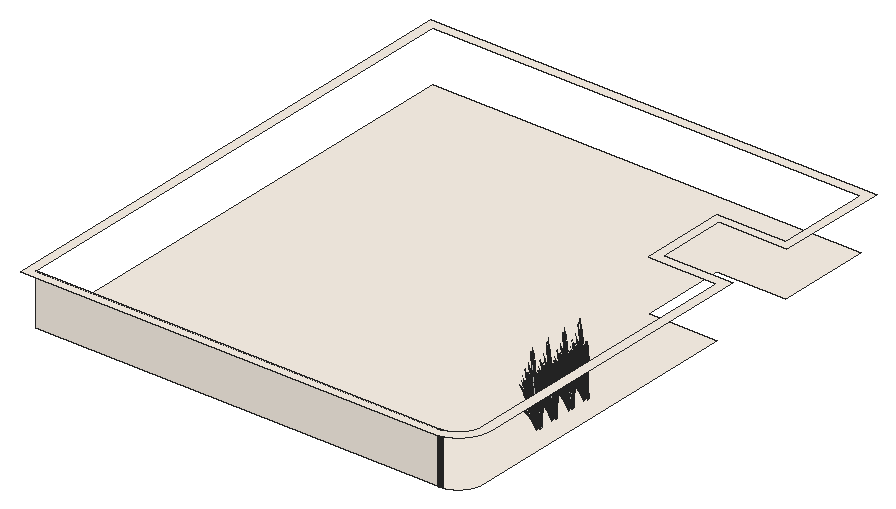
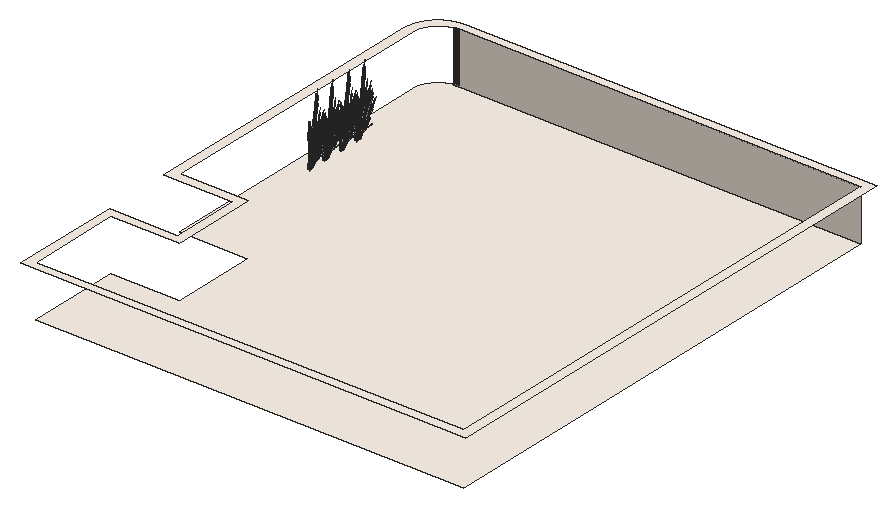
# SketchUp Ruby script. Lengths in inches.
U = 1.inch
M = Sketchup.active_model
def pt(a) = Geom::Point3d.new(a.map { |v| v * U })
def face(e, loops, mat)
  f = e.add_face(loops[0].map { |a| pt(a) })
  loops[1..].each { |l| e.add_face(l.map { |a| pt(a) }).erase! }
  f.material = f.back_material = mat if mat
  f
end
# faces: each face lists its corners as indices into pts; further lists are holes
def faces(e, pts, list, mat = nil) = list.each { |f| face(e, (f[0].is_a?(Array) ? f : [f]).map { |l| l.map { |i| pts[i] } }, mat) }
# xy, xz, yz: faces in a plane at the given z, y or x. An outline is a flat list of corners, or four numbers for a rectangle; further outlines are holes
def ring(l) = l.size == 4 ? [[l[0], l[1]], [l[2], l[1]], [l[2], l[3]], [l[0], l[3]]] : l.each_slice(2).to_a
def flat(e, list, mat, &to3) = list.each { |f| face(e, (f[0].is_a?(Array) ? f : [f]).map { |l| ring(l).map { |u, v| to3.(u, v) } }, mat) }
def xy(e, z, list, mat = nil) = flat(e, list, mat) { |x, y| [x, y, z] }
def xz(e, y, list, mat = nil) = flat(e, list, mat) { |x, z| [x, y, z] }
def yz(e, x, list, mat = nil) = flat(e, list, mat) { |y, z| [x, y, z] }
def lines(e, pts, list) = list.each { |a, b| e.add_line(pt(pts[a]), pt(pts[b])) }
# prism: a flat outline (further loops are holes) pulled along v
def prism(e, loops, v, mat = nil)
  f = face(e, loops, mat); d = Geom::Vector3d.new(v.map { |x| x * U })
  f.pushpull(f.normal.samedirection?(d) ? d.length : -d.length)
end
def box(e, o, s, mat = nil) = prism(e, [[o, [o[0] + s[0], o[1], o[2]], [o[0] + s[0], o[1] + s[1], o[2]], [o[0], o[1] + s[1], o[2]]]], [0, 0, s[2]], mat)
def at(x, y, z, deg = 0) = Geom::Transformation.translation(pt([x, y, z])) * Geom::Transformation.rotation(ORIGIN, Z_AXIS, deg.degrees)
def axes(o, x, y, z) = Geom::Transformation.new([*x, 0, *y, 0, *z, 0, *pt(o).to_a, 1])
def part(name) = M.definitions.add(name)
# library, detail: a bought-in or finely detailed component or shape, given as its bounding box
def library(name, o, s) = part(name).tap { |d| box(d.entities, o, s) }
def detail(e, o, s) = box(e.add_group.entities, o, s)
def put(e, d, t, mat = nil) = e.add_instance(d, t).tap { |i| i.material = mat if mat }
def group(e, t, mat = nil) = e.add_group.tap { |g| g.transformation = t; g.material = mat if mat }.entities
root = M.entities
M.materials.add("C01_Vanilla_Cream").color = [255, 246, 235]
M.materials.add("LightPink_Translucent").color = [144, 107, 117]
M.materials["LightPink_Translucent"].alpha = 0.75
c1 = part("blade")
p = [[2.15,0.21,22],[0,0.17,0],[0.09,0.45,0],[2.18,0.31,22],[2.29,0.31,22],[0.38,0.45,0],
  [2.48,0.24,33],[2.49,0.24,33],[2.48,0.22,33]]
faces(c1.entities,p,[[0,1,2,3],[4,5,2,3],[6,3,4,7],[8,0,3,6]])
c2 = part("seeds")
p = [[0.3,-0.1,1.38],[-0.01,-0.03,1.59],[-0.01,-0.03,0.03],[0.14,-0.07,-0.07],[0.29,-0.03,3],[0.15,0.01,3.11]]
faces(c2.entities,p,[[0,1,2,3],[1,0,4,5]],"LightPink_Translucent")
c3 = part("blade with seeds")
put(c3.entities,c1,at(0,0,0))
put(c3.entities,c2,axes([2.4,0.25,30.99],[1.5799,-0.05474,1.17369],[-0.12525,1.92788,0.29478],[-0.07173,-0.02425,1.56792]))
xy(root,654,[[54,12,336,12,336.57,12.01,337.13,12.04,337.69,12.08,338.26,12.14,338.82,12.22,339.37,12.32,339.93,12.43,340.48,12.57,341.02,12.71,341.5625,12.88,342.1,13.0625,342.625,13.26,343.15,13.48,343.66,13.71,344.17,13.96,344.67,14.23,345.16,14.51,345.64,14.8,346.12,15.11,346.58,15.4375,347.03,15.78,347.47,16.13,347.9,16.5,348.32,16.88,348.73,17.27,349.12,17.68,349.5,18.1,349.87,18.53,350.22,18.97,350.5625,19.42,350.89,19.88,351.2,20.36,351.49,20.84,351.77,21.33,352.04,21.83,352.29,22.34,352.52,22.85,352.74,23.375,352.9375,23.9,353.12,24.4375,353.29,24.98,353.43,25.52,353.57,26.07,353.68,26.63,353.78,27.18,353.86,27.74,353.92,28.31,353.96,28.87,353.99,29.43,354,30,354,234,306,234,306,294,354,294,354,360,54,360]],"C01_Vanilla_Cream")
xy(root,690,[[[48,6,336,6,336.75,6.01,337.51,6.05,338.26,6.11,339.01,6.1875,339.75,6.3,340.5,6.43,341.24,6.58,341.97,6.75,342.7,6.95,343.42,7.17,344.13,7.42,344.83,7.69,345.53,7.97,346.22,8.28,346.9,8.62,347.5625,8.97,348.22,9.34,348.86,9.74,349.49,10.15,350.11,10.58,350.71,11.04,351.3,11.51,351.87,12,352.43,12.5,352.97,13.03,353.5,13.57,354,14.13,354.49,14.7,354.96,15.29,355.42,15.89,355.85,16.51,356.26,17.14,356.66,17.78,357.03,18.4375,357.38,19.1,357.72,19.78,358.03,20.47,358.31,21.17,358.58,21.87,358.83,22.58,359.05,23.3,359.25,24.03,359.42,24.76,359.57,25.5,359.7,26.25,359.8125,26.99,359.89,27.74,359.95,28.49,359.99,29.25,360,30,360,240,312,240,312,288,360,288,360,366,48,366],[54,12,54,360,354,360,354,294,306,294,306,234,354,234,354,30,353.99,29.43,353.96,28.87,353.92,28.31,353.86,27.74,353.78,27.18,353.68,26.63,353.57,26.07,353.43,25.52,353.29,24.98,353.12,24.4375,352.9375,23.9,352.74,23.375,352.52,22.85,352.29,22.34,352.04,21.83,351.77,21.33,351.49,20.84,351.2,20.36,350.89,19.88,350.5625,19.42,350.22,18.97,349.87,18.53,349.5,18.1,349.12,17.68,348.73,17.27,348.32,16.88,347.9,16.5,347.47,16.13,347.03,15.78,346.58,15.4375,346.12,15.11,345.64,14.8,345.16,14.51,344.67,14.23,344.17,13.96,343.66,13.71,343.15,13.48,342.625,13.26,342.1,13.0625,341.5625,12.88,341.02,12.71,340.48,12.57,339.93,12.43,339.37,12.32,338.82,12.22,338.26,12.14,337.69,12.08,337.13,12.04,336.57,12.01,336,12]]],"C01_Vanilla_Cream")
xz(root,12,[[54,654,336,690]],"C01_Vanilla_Cream")
p = [[336.57,12.01,654],[336,12,654],[336,12,690],[336.57,12.01,690],[337.13,12.04,654],[337.13,12.04,690],
  [337.69,12.08,654],[337.69,12.08,690],[338.26,12.14,654],[338.26,12.14,690],[338.82,12.22,654],[338.82,12.22,690],
  [339.37,12.32,654],[339.37,12.32,690]]
faces(root,p,[[0,1,2,3],[4,0,3,5],[6,4,5,7],[8,6,7,9],[10,8,9,11],[12,10,11,13]],"C01_Vanilla_Cream")
put(root,c3,axes([339.83,94.1,657.18],[0.20495,-0.00938,1.40529],[-0.13596,0.40664,0.11363],[-0.29207,-0.02515,0.60075]))
put(root,c3,axes([339.83,107.7,657.18],[0.20495,-0.00938,1.40529],[-0.13596,0.40664,0.11363],[-0.29207,-0.02515,0.60075]))
put(root,c3,axes([339.83,122.09,657.18],[0.20495,-0.00938,1.40529],[-0.13596,0.40664,0.11363],[-0.29207,-0.02515,0.60075]))
put(root,c3,axes([339.83,135.58,657.18],[0.20495,-0.00938,1.40529],[-0.13596,0.40664,0.11363],[-0.29207,-0.02515,0.60075]))
put(root,c3,axes([339.92,94.81,657.18],[0.17145,-0.08763,1.40529],[0.14434,0.4049,0.11363],[-0.26915,0.09151,0.60075]))
put(root,c3,axes([339.92,108.41,657.18],[0.17145,-0.08763,1.40529],[0.14434,0.4049,0.11363],[-0.26915,0.09151,0.60075]))
put(root,c3,axes([339.92,122.81,657.18],[0.17145,-0.08763,1.40529],[0.14434,0.4049,0.11363],[-0.26915,0.09151,0.60075]))
put(root,c3,axes([339.92,136.3,657.18],[0.17145,-0.08763,1.40529],[0.14434,0.4049,0.11363],[-0.26915,0.09151,0.60075]))
put(root,c3,axes([339.39,95.5,656.125],[0.17172,0.03401,1.17261],[0.11068,0.34736,-0.25218],[-0.23326,0.06502,0.50135]))
put(root,c3,axes([339.39,109.1,656.125],[0.17172,0.03401,1.17261],[0.11068,0.34736,-0.25218],[-0.23326,0.06502,0.50135]))
put(root,c3,axes([339.39,123.5,656.125],[0.17172,0.03401,1.17261],[0.11068,0.34736,-0.25218],[-0.23326,0.06502,0.50135]))
put(root,c3,axes([339.39,136.99,656.125],[0.17172,0.03401,1.17261],[0.11068,0.34736,-0.25218],[-0.23326,0.06502,0.50135]))
put(root,c3,axes([340.9,94.39,656.74],[0.14045,-0.05993,1.45192],[0.04843,0.41842,0.11363],[-0.30422,0.05552,0.51893]))
put(root,c3,axes([340.9,107.99,656.74],[0.14045,-0.05993,1.45192],[0.04843,0.41842,0.11363],[-0.30422,0.05552,0.51893]))
put(root,c3,axes([340.9,122.39,656.74],[0.14045,-0.05993,1.45192],[0.04843,0.41842,0.11363],[-0.30422,0.05552,0.51893]))
put(root,c3,axes([340.9,135.875,656.74],[0.14045,-0.05993,1.45192],[0.04843,0.41842,0.11363],[-0.30422,0.05552,0.51893]))
put(root,c3,axes([339.39,94.67,657.87],[-0.08069,0.05378,1.43454],[0.00686,0.39297,-0.22687],[-0.18495,0.0511,0.11505]))
put(root,c3,axes([339.39,108.27,657.87],[-0.08069,0.05378,1.43454],[0.00686,0.39297,-0.22687],[-0.18495,0.0511,0.11505]))
put(root,c3,axes([339.39,122.67,657.87],[-0.08069,0.05378,1.43454],[0.00686,0.39297,-0.22687],[-0.18495,0.0511,0.11505]))
put(root,c3,axes([339.39,136.16,657.87],[-0.08069,0.05378,1.43454],[0.00686,0.39297,-0.22687],[-0.18495,0.0511,0.11505]))
put(root,c3,axes([340.45,93.72,658.08],[-0.49394,-0.00997,-0.58257],[0.03317,-0.42002,0.0703],[-0.20925,-0.04433,0.8241]))
put(root,c3,axes([340.45,107.32,658.08],[-0.49394,-0.00997,-0.58257],[0.03317,-0.42002,0.0703],[-0.20925,-0.04433,0.8241]))
put(root,c3,axes([340.45,121.72,658.08],[-0.49394,-0.00997,-0.58257],[0.03317,-0.42002,0.0703],[-0.20925,-0.04433,0.8241]))
put(root,c3,axes([340.45,135.21,658.08],[-0.49394,-0.00997,-0.58257],[0.03317,-0.42002,0.0703],[-0.20925,-0.04433,0.8241]))
put(root,c3,axes([340.05,93.82,656.125],[0.09647,0.11534,1.17261],[-0.2223,0.31351,-0.25218],[-0.22826,-0.07493,0.50135]))
put(root,c3,axes([340.05,107.42,656.125],[0.09647,0.11534,1.17261],[-0.2223,0.31351,-0.25218],[-0.22826,-0.07493,0.50135]))
put(root,c3,axes([340.05,121.82,656.125],[0.09647,0.11534,1.17261],[-0.2223,0.31351,-0.25218],[-0.22826,-0.07493,0.50135]))
put(root,c3,axes([340.05,135.31,656.125],[0.09647,0.11534,1.17261],[-0.2223,0.31351,-0.25218],[-0.22826,-0.07493,0.50135]))
put(root,c3,axes([339.65,94.45,657.71],[-0.41064,-0.11557,-0.29039],[0.11977,-0.33716,0.3749],[-0.16533,0.03092,0.71734]))
put(root,c3,axes([339.65,108.05,657.71],[-0.41064,-0.11557,-0.29039],[0.11977,-0.33716,0.3749],[-0.16533,0.03092,0.71734]))
put(root,c3,axes([339.65,122.44,657.71],[-0.41064,-0.11557,-0.29039],[0.11977,-0.33716,0.3749],[-0.16533,0.03092,0.71734]))
put(root,c3,axes([339.65,135.93,657.71],[-0.41064,-0.11557,-0.29039],[0.11977,-0.33716,0.3749],[-0.16533,0.03092,0.71734]))
put(root,c3,axes([340.22,93.45,657.18],[0.18354,0.07137,1.40529],[-0.37983,0.29943,0.11363],[-0.23673,-0.13508,0.60075]))
put(root,c3,axes([340.22,107.05,657.18],[0.18354,0.07137,1.40529],[-0.37983,0.29943,0.11363],[-0.23673,-0.13508,0.60075]))
put(root,c3,axes([340.22,121.44,657.18],[0.18354,0.07137,1.40529],[-0.37983,0.29943,0.11363],[-0.23673,-0.13508,0.60075]))
put(root,c3,axes([340.22,134.93,657.18],[0.18354,0.07137,1.40529],[-0.37983,0.29943,0.11363],[-0.23673,-0.13508,0.60075]))
put(root,c3,axes([338.5,95.07,657.86],[0.06306,0.01111,1.45454],[0.19508,0.36602,-0.13744],[-0.12909,0.09607,0.2574]))
put(root,c3,axes([338.5,108.67,657.86],[0.06306,0.01111,1.45454],[0.19508,0.36602,-0.13744],[-0.12909,0.09607,0.2574]))
put(root,c3,axes([338.5,123.0625,657.86],[0.06306,0.01111,1.45454],[0.19508,0.36602,-0.13744],[-0.12909,0.09607,0.2574]))
put(root,c3,axes([338.5,136.55,657.86],[0.06306,0.01111,1.45454],[0.19508,0.36602,-0.13744],[-0.12909,0.09607,0.2574]))
put(root,c3,axes([339.94,94.62,657.84],[-0.13386,0.37682,-0.41901],[-0.45895,-0.12916,-0.32456],[-0.18478,0.03455,0.80174]))
put(root,c3,axes([339.94,108.22,657.84],[-0.13386,0.37682,-0.41901],[-0.45895,-0.12916,-0.32456],[-0.18478,0.03455,0.80174]))
put(root,c3,axes([339.94,122.61,657.84],[-0.13386,0.37682,-0.41901],[-0.45895,-0.12916,-0.32456],[-0.18478,0.03455,0.80174]))
put(root,c3,axes([339.94,136.1,657.84],[-0.13386,0.37682,-0.41901],[-0.45895,-0.12916,-0.32456],[-0.18478,0.03455,0.80174]))
put(root,c3,axes([340.28,93.81,657.84],[-0.35879,0.27441,-0.41901],[-0.31422,-0.28988,-0.32456],[-0.18229,-0.04175,0.80174]))
put(root,c3,axes([340.28,107.4,657.84],[-0.35879,0.27441,-0.41901],[-0.31422,-0.28988,-0.32456],[-0.18229,-0.04175,0.80174]))
put(root,c3,axes([340.28,121.8,657.84],[-0.35879,0.27441,-0.41901],[-0.31422,-0.28988,-0.32456],[-0.18229,-0.04175,0.80174]))
put(root,c3,axes([340.28,135.29,657.84],[-0.35879,0.27441,-0.41901],[-0.31422,-0.28988,-0.32456],[-0.18229,-0.04175,0.80174]))
put(root,c3,axes([339.7,94.6,655.22],[0.01253,0.06529,1.44601],[-0.25262,0.34095,-0.2209],[-0.17944,-0.01719,0.2463]))
put(root,c3,axes([339.7,108.2,655.22],[0.01253,0.06529,1.44601],[-0.25262,0.34095,-0.2209],[-0.17944,-0.01719,0.2463]))
put(root,c3,axes([339.7,122.59,655.22],[0.01253,0.06529,1.44601],[-0.25262,0.34095,-0.2209],[-0.17944,-0.01719,0.2463]))
put(root,c3,axes([339.7,136.08,655.22],[0.01253,0.06529,1.44601],[-0.25262,0.34095,-0.2209],[-0.17944,-0.01719,0.2463]))
put(root,c3,axes([339.78,93.04,657.86],[0.03663,0.04134,1.45454],[-0.17659,0.37163,-0.13744],[-0.17885,0.00269,0.2574]))
put(root,c3,axes([339.78,106.64,657.86],[0.03663,0.04134,1.45454],[-0.17659,0.37163,-0.13744],[-0.17885,0.00269,0.2574]))
put(root,c3,axes([339.78,121.03,657.86],[0.03663,0.04134,1.45454],[-0.17659,0.37163,-0.13744],[-0.17885,0.00269,0.2574]))
put(root,c3,axes([339.78,134.52,657.86],[0.03663,0.04134,1.45454],[-0.17659,0.37163,-0.13744],[-0.17885,0.00269,0.2574]))
put(root,c3,axes([339.03,96.23,656.27],[0.20592,-0.18775,0.94186],[0.08126,0.29723,0.69201],[-0.14881,0.05322,0.20745]))
put(root,c3,axes([339.03,109.83,656.27],[0.20592,-0.18775,0.94186],[0.08126,0.29723,0.69201],[-0.14881,0.05322,0.20745]))
put(root,c3,axes([339.03,124.23,656.27],[0.20592,-0.18775,0.94186],[0.08126,0.29723,0.69201],[-0.14881,0.05322,0.20745]))
put(root,c3,axes([339.03,137.72,656.27],[0.20592,-0.18775,0.94186],[0.08126,0.29723,0.69201],[-0.14881,0.05322,0.20745]))
put(root,c3,axes([340.1875,92.79,657.87],[-0.10632,-0.00292,1.43454],[-0.33847,0.29241,-0.22687],[-0.1806,-0.05975,0.11505]))
put(root,c3,axes([340.1875,106.39,657.87],[-0.10632,-0.00292,1.43454],[-0.33847,0.29241,-0.22687],[-0.1806,-0.05975,0.11505]))
put(root,c3,axes([340.1875,120.78,657.87],[-0.10632,-0.00292,1.43454],[-0.33847,0.29241,-0.22687],[-0.1806,-0.05975,0.11505]))
put(root,c3,axes([340.1875,134.27,657.87],[-0.10632,-0.00292,1.43454],[-0.33847,0.29241,-0.22687],[-0.1806,-0.05975,0.11505]))
put(root,c3,axes([339.75,94.41,657.88],[0.1396,-0.37772,0.39362],[0.45895,0.12916,0.32456],[-0.18049,0.0227,0.8145]))
put(root,c3,axes([339.75,108.01,657.88],[0.1396,-0.37772,0.39362],[0.45895,0.12916,0.32456],[-0.18049,0.0227,0.8145]))
put(root,c3,axes([339.75,122.4,657.88],[0.1396,-0.37772,0.39362],[0.45895,0.12916,0.32456],[-0.18049,0.0227,0.8145]))
put(root,c3,axes([339.75,135.89,657.88],[0.1396,-0.37772,0.39362],[0.45895,0.12916,0.32456],[-0.18049,0.0227,0.8145]))
put(root,c3,axes([339.91,94.3,658.13],[0.24861,0.37512,-0.09971],[-0.44125,0.18434,-0.55346],[-0.18594,0.04949,0.84097]))
put(root,c3,axes([339.91,107.9,658.13],[0.24861,0.37512,-0.09971],[-0.44125,0.18434,-0.55346],[-0.18594,0.04949,0.84097]))
put(root,c3,axes([339.91,122.29,658.13],[0.24861,0.37512,-0.09971],[-0.44125,0.18434,-0.55346],[-0.18594,0.04949,0.84097]))
put(root,c3,axes([339.91,135.78,658.13],[0.24861,0.37512,-0.09971],[-0.44125,0.18434,-0.55346],[-0.18594,0.04949,0.84097]))
put(root,c3,axes([340.47,93.52,658.13],[-0.02646,0.4213,-0.09971],[-0.50094,-0.01152,-0.55346],[-0.19293,-0.02926,0.84097]))
put(root,c3,axes([340.47,107.12,658.13],[-0.02646,0.4213,-0.09971],[-0.50094,-0.01152,-0.55346],[-0.19293,-0.02926,0.84097]))
put(root,c3,axes([340.47,121.51,658.13],[-0.02646,0.4213,-0.09971],[-0.50094,-0.01152,-0.55346],[-0.19293,-0.02926,0.84097]))
put(root,c3,axes([340.47,135,658.13],[-0.02646,0.4213,-0.09971],[-0.50094,-0.01152,-0.55346],[-0.19293,-0.02926,0.84097]))
put(root,c3,axes([340.15,93.55,657.71],[-0.28114,-0.25937,-0.29039],[0.32102,-0.24553,0.3749],[-0.16311,-0.03736,0.71734]))
put(root,c3,axes([340.15,107.15,657.71],[-0.28114,-0.25937,-0.29039],[0.32102,-0.24553,0.3749],[-0.16311,-0.03736,0.71734]))
put(root,c3,axes([340.15,121.54,657.71],[-0.28114,-0.25937,-0.29039],[0.32102,-0.24553,0.3749],[-0.16311,-0.03736,0.71734]))
put(root,c3,axes([340.15,135.03,657.71],[-0.28114,-0.25937,-0.29039],[0.32102,-0.24553,0.3749],[-0.16311,-0.03736,0.71734]))
put(root,c3,axes([339.71,94.31,657.88],[-0.18148,-0.28246,0.05273],[0.33093,-0.13825,0.41509],[-0.14588,0.02728,0.63295]))
put(root,c3,axes([339.71,107.9,657.88],[-0.18148,-0.28246,0.05273],[0.33093,-0.13825,0.41509],[-0.14588,0.02728,0.63295]))
put(root,c3,axes([339.71,122.3,657.88],[-0.18148,-0.28246,0.05273],[0.33093,-0.13825,0.41509],[-0.14588,0.02728,0.63295]))
put(root,c3,axes([339.71,135.79,657.88],[-0.18148,-0.28246,0.05273],[0.33093,-0.13825,0.41509],[-0.14588,0.02728,0.63295]))
put(root,c3,axes([340.55,95.09,657.18],[0.12341,-0.12729,1.40529],[0.31162,0.34357,0.11363],[-0.21373,0.15646,0.60075]))
put(root,c3,axes([340.55,108.6875,657.18],[0.12341,-0.12729,1.40529],[0.31162,0.34357,0.11363],[-0.21373,0.15646,0.60075]))
put(root,c3,axes([340.55,123.08,657.18],[0.12341,-0.12729,1.40529],[0.31162,0.34357,0.11363],[-0.21373,0.15646,0.60075]))
put(root,c3,axes([340.55,136.57,657.18],[0.12341,-0.12729,1.40529],[0.31162,0.34357,0.11363],[-0.21373,0.15646,0.60075]))
put(root,c3,axes([339.8,95.42,657.71],[-0.43011,0.0592,-0.29039],[-0.11357,-0.33844,0.3749],[-0.12326,0.0909,0.71734]))
put(root,c3,axes([339.8,109.02,657.71],[-0.43011,0.0592,-0.29039],[-0.11357,-0.33844,0.3749],[-0.12326,0.0909,0.71734]))
put(root,c3,axes([339.8,123.41,657.71],[-0.43011,0.0592,-0.29039],[-0.11357,-0.33844,0.3749],[-0.12326,0.0909,0.71734]))
put(root,c3,axes([339.8,136.91,657.71],[-0.43011,0.0592,-0.29039],[-0.11357,-0.33844,0.3749],[-0.12326,0.0909,0.71734]))
put(root,c3,axes([339.57,96.43,655.22],[0.06628,0.04139,1.44601],[0.11238,0.38347,-0.2209],[-0.14689,0.08177,0.2463]))
put(root,c3,axes([339.57,110.02,655.22],[0.06628,0.04139,1.44601],[0.11238,0.38347,-0.2209],[-0.14689,0.08177,0.2463]))
put(root,c3,axes([339.57,124.42,655.22],[0.06628,0.04139,1.44601],[0.11238,0.38347,-0.2209],[-0.14689,0.08177,0.2463]))
put(root,c3,axes([339.57,137.91,655.22],[0.06628,0.04139,1.44601],[0.11238,0.38347,-0.2209],[-0.14689,0.08177,0.2463]))
put(root,c3,axes([339.47,94.17,656.27],[0.31546,-0.02964,0.94186],[-0.20011,0.26119,0.69201],[-0.15589,-0.03918,0.20745]))
put(root,c3,axes([339.47,107.77,656.27],[0.31546,-0.02964,0.94186],[-0.20011,0.26119,0.69201],[-0.15589,-0.03918,0.20745]))
put(root,c3,axes([339.47,122.16,656.27],[0.31546,-0.02964,0.94186],[-0.20011,0.26119,0.69201],[-0.15589,-0.03918,0.20745]))
put(root,c3,axes([339.47,135.65,656.27],[0.31546,-0.02964,0.94186],[-0.20011,0.26119,0.69201],[-0.15589,-0.03918,0.20745]))
put(root,c3,axes([339.86,95.35,657.88],[-0.12254,-0.38127,0.39362],[0.48071,-0.06617,0.32456],[-0.14168,0.08967,0.8145]))
put(root,c3,axes([339.86,108.95,657.88],[-0.12254,-0.38127,0.39362],[0.48071,-0.06617,0.32456],[-0.14168,0.08967,0.8145]))
put(root,c3,axes([339.86,123.34,657.88],[-0.12254,-0.38127,0.39362],[0.48071,-0.06617,0.32456],[-0.14168,0.08967,0.8145]))
put(root,c3,axes([339.86,136.83,657.88],[-0.12254,-0.38127,0.39362],[0.48071,-0.06617,0.32456],[-0.14168,0.08967,0.8145]))
put(root,c3,axes([340.11,93.45,658.18],[0.40806,-0.30572,0.44086],[0.35193,0.32467,0.3635],[-0.19145,-0.05639,0.91224]))
put(root,c3,axes([340.11,107.05,658.18],[0.40806,-0.30572,0.44086],[0.35193,0.32467,0.3635],[-0.19145,-0.05639,0.91224]))
put(root,c3,axes([340.11,121.44,658.18],[0.40806,-0.30572,0.44086],[0.35193,0.32467,0.3635],[-0.19145,-0.05639,0.91224]))
put(root,c3,axes([340.11,134.94,658.18],[0.40806,-0.30572,0.44086],[0.35193,0.32467,0.3635],[-0.19145,-0.05639,0.91224]))
put(root,c3,axes([339.76,95.27,657.88],[-0.33921,-0.17422,0.05273],[0.19749,-0.2481,0.41509],[-0.10876,0.08021,0.63295]))
put(root,c3,axes([339.76,108.87,657.88],[-0.33921,-0.17422,0.05273],[0.19749,-0.2481,0.41509],[-0.10876,0.08021,0.63295]))
put(root,c3,axes([339.76,123.27,657.88],[-0.33921,-0.17422,0.05273],[0.19749,-0.2481,0.41509],[-0.10876,0.08021,0.63295]))
put(root,c3,axes([339.76,136.76,657.88],[-0.33921,-0.17422,0.05273],[0.19749,-0.2481,0.41509],[-0.10876,0.08021,0.63295]))
put(root,c3,axes([340.45,95.4,657.18],[0.092,-0.14239,1.40529],[0.38596,0.29467,0.11363],[-0.17411,0.18366,0.60075]))
put(root,c3,axes([340.45,109,657.18],[0.092,-0.14239,1.40529],[0.38596,0.29467,0.11363],[-0.17411,0.18366,0.60075]))
put(root,c3,axes([340.45,123.4,657.18],[0.092,-0.14239,1.40529],[0.38596,0.29467,0.11363],[-0.17411,0.18366,0.60075]))
put(root,c3,axes([340.09,94.41,658.14],[0.41064,0.11557,0.29039],[-0.11977,0.33716,-0.3749],[-0.16533,0.03092,0.71734]))
put(root,c3,axes([340.09,108.01,658.14],[0.41064,0.11557,0.29039],[-0.11977,0.33716,-0.3749],[-0.16533,0.03092,0.71734]))
put(root,c3,axes([340.09,122.41,658.14],[0.41064,0.11557,0.29039],[-0.11977,0.33716,-0.3749],[-0.16533,0.03092,0.71734]))
put(root,c3,axes([340.09,135.9,658.14],[0.41064,0.11557,0.29039],[-0.11977,0.33716,-0.3749],[-0.16533,0.03092,0.71734]))
put(root,c3,axes([340.16,95.46,657.84],[0.12693,0.37826,-0.41901],[-0.48071,0.06617,-0.32456],[-0.13776,0.1016,0.80174]))
put(root,c3,axes([340.16,109.06,657.84],[0.12693,0.37826,-0.41901],[-0.48071,0.06617,-0.32456],[-0.13776,0.1016,0.80174]))
put(root,c3,axes([340.16,123.45,657.84],[0.12693,0.37826,-0.41901],[-0.48071,0.06617,-0.32456],[-0.13776,0.1016,0.80174]))
put(root,c3,axes([340.16,136.94,657.84],[0.12693,0.37826,-0.41901],[-0.48071,0.06617,-0.32456],[-0.13776,0.1016,0.80174]))
put(root,c3,axes([340.29,93.45,657.88],[0.02488,-0.31501,0.05273],[0.3757,0.00864,0.41509],[-0.14392,-0.03296,0.63295]))
put(root,c3,axes([340.29,107.05,657.88],[0.02488,-0.31501,0.05273],[0.3757,0.00864,0.41509],[-0.14392,-0.03296,0.63295]))
put(root,c3,axes([340.29,121.44,657.88],[0.02488,-0.31501,0.05273],[0.3757,0.00864,0.41509],[-0.14392,-0.03296,0.63295]))
put(root,c3,axes([340.29,134.93,657.88],[0.02488,-0.31501,0.05273],[0.3757,0.00864,0.41509],[-0.14392,-0.03296,0.63295]))
put(root,c3,axes([339.41,96.14,657.87],[-0.01228,0.08198,1.43454],[0.34856,0.28519,-0.22687],[-0.09125,0.13486,0.11505]))
put(root,c3,axes([339.41,109.74,657.87],[-0.01228,0.08198,1.43454],[0.34856,0.28519,-0.22687],[-0.09125,0.13486,0.11505]))
put(root,c3,axes([339.41,124.13,657.87],[-0.01228,0.08198,1.43454],[0.34856,0.28519,-0.22687],[-0.09125,0.13486,0.11505]))
put(root,c3,axes([341.36,95.1875,655.6875],[-0.514,-0.06792,-0.51129],[0.10846,-0.41895,-0.13419],[-0.15339,-0.05076,1.12859]))
put(root,c3,axes([341.36,108.79,655.6875],[-0.514,-0.06792,-0.51129],[0.10846,-0.41895,-0.13419],[-0.15339,-0.05076,1.12859]))
put(root,c3,axes([341.36,123.18,655.6875],[-0.514,-0.06792,-0.51129],[0.10846,-0.41895,-0.13419],[-0.15339,-0.05076,1.12859]))
put(root,c3,axes([341.36,136.67,655.6875],[-0.514,-0.06792,-0.51129],[0.10846,-0.41895,-0.13419],[-0.15339,-0.05076,1.12859]))
put(root,c3,axes([341.45,92.9,658.45],[-0.32977,0.39714,-0.11168],[-0.47757,-0.2288,-0.61987],[-0.16601,-0.1122,0.94188]))
put(root,c3,axes([341.45,106.5,658.45],[-0.32977,0.39714,-0.11168],[-0.47757,-0.2288,-0.61987],[-0.16601,-0.1122,0.94188]))
put(root,c3,axes([341.45,120.9,658.45],[-0.32977,0.39714,-0.11168],[-0.47757,-0.2288,-0.61987],[-0.16601,-0.1122,0.94188]))
put(root,c3,axes([341.45,134.39,658.45],[-0.32977,0.39714,-0.11168],[-0.47757,-0.2288,-0.61987],[-0.16601,-0.1122,0.94188]))
put(root,c3,axes([340.55,93.68,658.14],[0.28114,0.25937,0.29039],[-0.32102,0.24553,-0.3749],[-0.16311,-0.03736,0.71734]))
put(root,c3,axes([340.55,107.28,658.14],[0.28114,0.25937,0.29039],[-0.32102,0.24553,-0.3749],[-0.16311,-0.03736,0.71734]))
put(root,c3,axes([340.55,121.68,658.14],[0.28114,0.25937,0.29039],[-0.32102,0.24553,-0.3749],[-0.16311,-0.03736,0.71734]))
put(root,c3,axes([340.55,135.17,658.14],[0.28114,0.25937,0.29039],[-0.32102,0.24553,-0.3749],[-0.16311,-0.03736,0.71734]))
put(root,c3,axes([341.31,93.23,658.08],[-0.42133,-0.20023,-0.58257],[0.29943,-0.35088,0.0703],[-0.15265,-0.11956,0.8241]))
put(root,c3,axes([341.31,106.82,658.08],[-0.42133,-0.20023,-0.58257],[0.29943,-0.35088,0.0703],[-0.15265,-0.11956,0.8241]))
put(root,c3,axes([341.31,121.22,658.08],[-0.42133,-0.20023,-0.58257],[0.29943,-0.35088,0.0703],[-0.15265,-0.11956,0.8241]))
put(root,c3,axes([341.31,134.71,658.08],[-0.42133,-0.20023,-0.58257],[0.29943,-0.35088,0.0703],[-0.15265,-0.11956,0.8241]))
put(root,c3,axes([341.11,93.24,657.84],[-0.48758,0.09847,-0.41901],[-0.08529,-0.37293,-0.32456],[-0.13096,-0.10687,0.80174]))
put(root,c3,axes([341.11,106.83,657.84],[-0.48758,0.09847,-0.41901],[-0.08529,-0.37293,-0.32456],[-0.13096,-0.10687,0.80174]))
put(root,c3,axes([341.11,121.23,657.84],[-0.48758,0.09847,-0.41901],[-0.08529,-0.37293,-0.32456],[-0.13096,-0.10687,0.80174]))
put(root,c3,axes([341.11,134.72,657.84],[-0.48758,0.09847,-0.41901],[-0.08529,-0.37293,-0.32456],[-0.13096,-0.10687,0.80174]))
put(root,c3,axes([340.68,95.98,655.65],[-0.46245,-0.20713,-0.40713],[0.27641,-0.37142,0],[-0.10533,-0.04718,1.29153]))
put(root,c3,axes([340.68,109.58,655.65],[-0.46245,-0.20713,-0.40713],[0.27641,-0.37142,0],[-0.10533,-0.04718,1.29153]))
put(root,c3,axes([340.68,123.98,655.65],[-0.46245,-0.20713,-0.40713],[0.27641,-0.37142,0],[-0.10533,-0.04718,1.29153]))
put(root,c3,axes([340.68,137.47,655.65],[-0.46245,-0.20713,-0.40713],[0.27641,-0.37142,0],[-0.10533,-0.04718,1.29153]))
put(root,c3,axes([340.48,92.9,655.22],[-0.04786,0.05457,1.44601],[-0.48369,0.11766,-0.2209],[-0.11685,-0.10703,0.2463]))
put(root,c3,axes([340.48,106.5,655.22],[-0.04786,0.05457,1.44601],[-0.48369,0.11766,-0.2209],[-0.11685,-0.10703,0.2463]))
put(root,c3,axes([340.48,120.89,655.22],[-0.04786,0.05457,1.44601],[-0.48369,0.11766,-0.2209],[-0.11685,-0.10703,0.2463]))
put(root,c3,axes([340.48,134.38,655.22],[-0.04786,0.05457,1.44601],[-0.48369,0.11766,-0.2209],[-0.11685,-0.10703,0.2463]))
put(root,c3,axes([339.93,95.19,658.13],[0.45707,0.22842,-0.09971],[-0.26332,0.3308,-0.55346],[-0.12913,0.11499,0.84097]))
put(root,c3,axes([339.93,108.79,658.13],[0.45707,0.22842,-0.09971],[-0.26332,0.3308,-0.55346],[-0.12913,0.11499,0.84097]))
put(root,c3,axes([339.93,123.18,658.13],[0.45707,0.22842,-0.09971],[-0.26332,0.3308,-0.55346],[-0.12913,0.11499,0.84097]))
put(root,c3,axes([339.93,136.67,658.13],[0.45707,0.22842,-0.09971],[-0.26332,0.3308,-0.55346],[-0.12913,0.11499,0.84097]))
put(root,c3,axes([340.96,96.23,655.95],[-0.30893,0.41511,0],[-0.51685,-0.2315,-0.42318],[-0.11772,-0.05273,1.34243]))
put(root,c3,axes([340.96,109.83,655.95],[-0.30893,0.41511,0],[-0.51685,-0.2315,-0.42318],[-0.11772,-0.05273,1.34243]))
put(root,c3,axes([340.96,124.23,655.95],[-0.30893,0.41511,0],[-0.51685,-0.2315,-0.42318],[-0.11772,-0.05273,1.34243]))
put(root,c3,axes([340.96,137.72,655.95],[-0.30893,0.41511,0],[-0.51685,-0.2315,-0.42318],[-0.11772,-0.05273,1.34243]))
put(root,c3,axes([339.18,96.18,658.63],[0.43603,0.11058,-0.0532],[-0.13413,0.34034,-0.24121],[-0.07132,0.05167,0.7956]))
put(root,c3,axes([339.18,109.78,658.63],[0.43603,0.11058,-0.0532],[-0.13413,0.34034,-0.24121],[-0.07132,0.05167,0.7956]))
put(root,c3,axes([339.18,124.18,658.63],[0.43603,0.11058,-0.0532],[-0.13413,0.34034,-0.24121],[-0.07132,0.05167,0.7956]))
put(root,c3,axes([339.18,137.67,658.63],[0.43603,0.11058,-0.0532],[-0.13413,0.34034,-0.24121],[-0.07132,0.05167,0.7956]))
put(root,c3,axes([340.15,95.22,658.14],[0.43011,-0.0592,0.29039],[0.11357,0.33844,-0.3749],[-0.12326,0.0909,0.71734]))
put(root,c3,axes([340.15,108.82,658.14],[0.43011,-0.0592,0.29039],[0.11357,0.33844,-0.3749],[-0.12326,0.0909,0.71734]))
put(root,c3,axes([340.15,123.21,658.14],[0.43011,-0.0592,0.29039],[0.11357,0.33844,-0.3749],[-0.12326,0.0909,0.71734]))
put(root,c3,axes([340.15,136.71,658.14],[0.43011,-0.0592,0.29039],[0.11357,0.33844,-0.3749],[-0.12326,0.0909,0.71734]))
put(root,c3,axes([340.4,96.83,656.125],[0.15593,-0.06535,1.17261],[0.38498,0.19705,-0.25218],[-0.11459,0.1705,0.50135]))
put(root,c3,axes([340.4,110.43,656.125],[0.15593,-0.06535,1.17261],[0.38498,0.19705,-0.25218],[-0.11459,0.1705,0.50135]))
put(root,c3,axes([340.4,124.83,656.125],[0.15593,-0.06535,1.17261],[0.38498,0.19705,-0.25218],[-0.11459,0.1705,0.50135]))
put(root,c3,axes([340.18,93.11,655.74],[-0.14254,0.33827,-0.03192],[-0.4387,-0.10405,-0.14473],[-0.06661,-0.05533,0.47736]))
put(root,c3,axes([340.18,106.71,655.74],[-0.14254,0.33827,-0.03192],[-0.4387,-0.10405,-0.14473],[-0.06661,-0.05533,0.47736]))
put(root,c3,axes([340.18,121.1,655.74],[-0.14254,0.33827,-0.03192],[-0.4387,-0.10405,-0.14473],[-0.06661,-0.05533,0.47736]))
put(root,c3,axes([340.18,134.59,655.74],[-0.14254,0.33827,-0.03192],[-0.4387,-0.10405,-0.14473],[-0.06661,-0.05533,0.47736]))
put(root,c3,axes([341.32,91.96,657.86],[-0.00922,0.04965,1.45454],[-0.45464,0.18021,-0.13744],[-0.13379,-0.09212,0.2574]))
put(root,c3,axes([341.32,105.56,657.86],[-0.00922,0.04965,1.45454],[-0.45464,0.18021,-0.13744],[-0.13379,-0.09212,0.2574]))
put(root,c3,axes([341.32,119.95,657.86],[-0.00922,0.04965,1.45454],[-0.45464,0.18021,-0.13744],[-0.13379,-0.09212,0.2574]))
put(root,c3,axes([341.32,133.44,657.86],[-0.00922,0.04965,1.45454],[-0.45464,0.18021,-0.13744],[-0.13379,-0.09212,0.2574]))
put(root,c3,axes([340.83,92.68,656.125],[-0.02992,0.13552,1.17261],[-0.43742,0.11344,-0.25218],[-0.10225,-0.17516,0.50135]))
put(root,c3,axes([340.83,106.28,656.125],[-0.02992,0.13552,1.17261],[-0.43742,0.11344,-0.25218],[-0.10225,-0.17516,0.50135]))
put(root,c3,axes([340.83,120.67,656.125],[-0.02992,0.13552,1.17261],[-0.43742,0.11344,-0.25218],[-0.10225,-0.17516,0.50135]))
put(root,c3,axes([340.83,134.16,656.125],[-0.02992,0.13552,1.17261],[-0.43742,0.11344,-0.25218],[-0.10225,-0.17516,0.50135]))
put(root,c3,axes([340.98,93.03,657.18],[0.11295,0.13301,1.40529],[-0.52192,0.11198,0.11363],[-0.11796,-0.20881,0.60075]))
put(root,c3,axes([340.98,106.63,657.18],[0.11295,0.13301,1.40529],[-0.52192,0.11198,0.11363],[-0.11796,-0.20881,0.60075]))
put(root,c3,axes([340.98,121.03,657.18],[0.11295,0.13301,1.40529],[-0.52192,0.11198,0.11363],[-0.11796,-0.20881,0.60075]))
put(root,c3,axes([340.98,134.52,657.18],[0.11295,0.13301,1.40529],[-0.52192,0.11198,0.11363],[-0.11796,-0.20881,0.60075]))
put(root,c3,axes([341.94,95.25,656.1875],[-0.49889,0.27503,-0.23858],[-0.33175,-0.38862,-0.41002],[-0.12309,-0.03947,1.3096]))
put(root,c3,axes([341.94,108.85,656.1875],[-0.49889,0.27503,-0.23858],[-0.33175,-0.38862,-0.41002],[-0.12309,-0.03947,1.3096]))
put(root,c3,axes([341.94,123.24,656.1875],[-0.49889,0.27503,-0.23858],[-0.33175,-0.38862,-0.41002],[-0.12309,-0.03947,1.3096]))
put(root,c3,axes([341.94,136.74,656.1875],[-0.49889,0.27503,-0.23858],[-0.33175,-0.38862,-0.41002],[-0.12309,-0.03947,1.3096]))
put(root,c3,axes([340.5625,96.12,657.88],[-0.35185,-0.28265,0.39362],[0.37366,-0.24377,0.32456],[-0.0649,0.13261,0.8145]))
put(root,c3,axes([340.5625,109.72,657.88],[-0.35185,-0.28265,0.39362],[0.37366,-0.24377,0.32456],[-0.0649,0.13261,0.8145]))
put(root,c3,axes([340.5625,124.11,657.88],[-0.35185,-0.28265,0.39362],[0.37366,-0.24377,0.32456],[-0.0649,0.13261,0.8145]))
put(root,c3,axes([340.5625,137.6,657.88],[-0.35185,-0.28265,0.39362],[0.37366,-0.24377,0.32456],[-0.0649,0.13261,0.8145]))
put(root,c3,axes([341.16,92.96,657.71],[-0.07631,-0.33368,-0.29039],[0.43626,-0.08811,0.3749],[-0.11718,-0.09562,0.71734]))
put(root,c3,axes([341.16,106.56,657.71],[-0.07631,-0.33368,-0.29039],[0.43626,-0.08811,0.3749],[-0.11718,-0.09562,0.71734]))
put(root,c3,axes([341.16,120.96,657.71],[-0.07631,-0.33368,-0.29039],[0.43626,-0.08811,0.3749],[-0.11718,-0.09562,0.71734]))
put(root,c3,axes([341.16,134.45,657.71],[-0.07631,-0.33368,-0.29039],[0.43626,-0.08811,0.3749],[-0.11718,-0.09562,0.71734]))
put(root,c3,axes([339.94,94.65,655.95],[-0.61786,0,0],[0,-0.463,-0.42318],[0,-0.10545,1.34243]))
put(root,c3,axes([339.94,108.25,655.95],[-0.61786,0,0],[0,-0.463,-0.42318],[0,-0.10545,1.34243]))
put(root,c3,axes([339.94,122.64,655.95],[-0.61786,0,0],[0,-0.463,-0.42318],[0,-0.10545,1.34243]))
put(root,c3,axes([339.94,136.14,655.95],[-0.61786,0,0],[0,-0.463,-0.42318],[0,-0.10545,1.34243]))
put(root,c3,axes([340.8125,95.83,655.66],[-0.11607,-0.36097,-0.25402],[0.46099,-0.1025,0.25402],[-0.09293,-0.04163,1.13959]))
put(root,c3,axes([340.8125,109.43,655.66],[-0.11607,-0.36097,-0.25402],[0.46099,-0.1025,0.25402],[-0.09293,-0.04163,1.13959]))
put(root,c3,axes([340.8125,123.82,655.66],[-0.11607,-0.36097,-0.25402],[0.46099,-0.1025,0.25402],[-0.09293,-0.04163,1.13959]))
put(root,c3,axes([340.8125,137.3125,655.66],[-0.11607,-0.36097,-0.25402],[0.46099,-0.1025,0.25402],[-0.09293,-0.04163,1.13959]))
put(root,c3,axes([340.43,96.09,657.88],[-0.40605,-0.0193,0.05273],[0.01113,-0.29147,0.41509],[-0.04249,0.11165,0.63295]))
put(root,c3,axes([340.43,109.69,657.88],[-0.40605,-0.0193,0.05273],[0.01113,-0.29147,0.41509],[-0.04249,0.11165,0.63295]))
put(root,c3,axes([340.43,124.09,657.88],[-0.40605,-0.0193,0.05273],[0.01113,-0.29147,0.41509],[-0.04249,0.11165,0.63295]))
put(root,c3,axes([340.43,137.58,657.88],[-0.40605,-0.0193,0.05273],[0.01113,-0.29147,0.41509],[-0.04249,0.11165,0.63295]))
put(root,c3,axes([340.5625,96.2,657.71],[-0.33433,0.21811,-0.29039],[-0.31649,-0.24905,0.3749],[-0.04815,0.12654,0.71734]))
put(root,c3,axes([340.5625,109.8,657.71],[-0.33433,0.21811,-0.29039],[-0.31649,-0.24905,0.3749],[-0.04815,0.12654,0.71734]))
